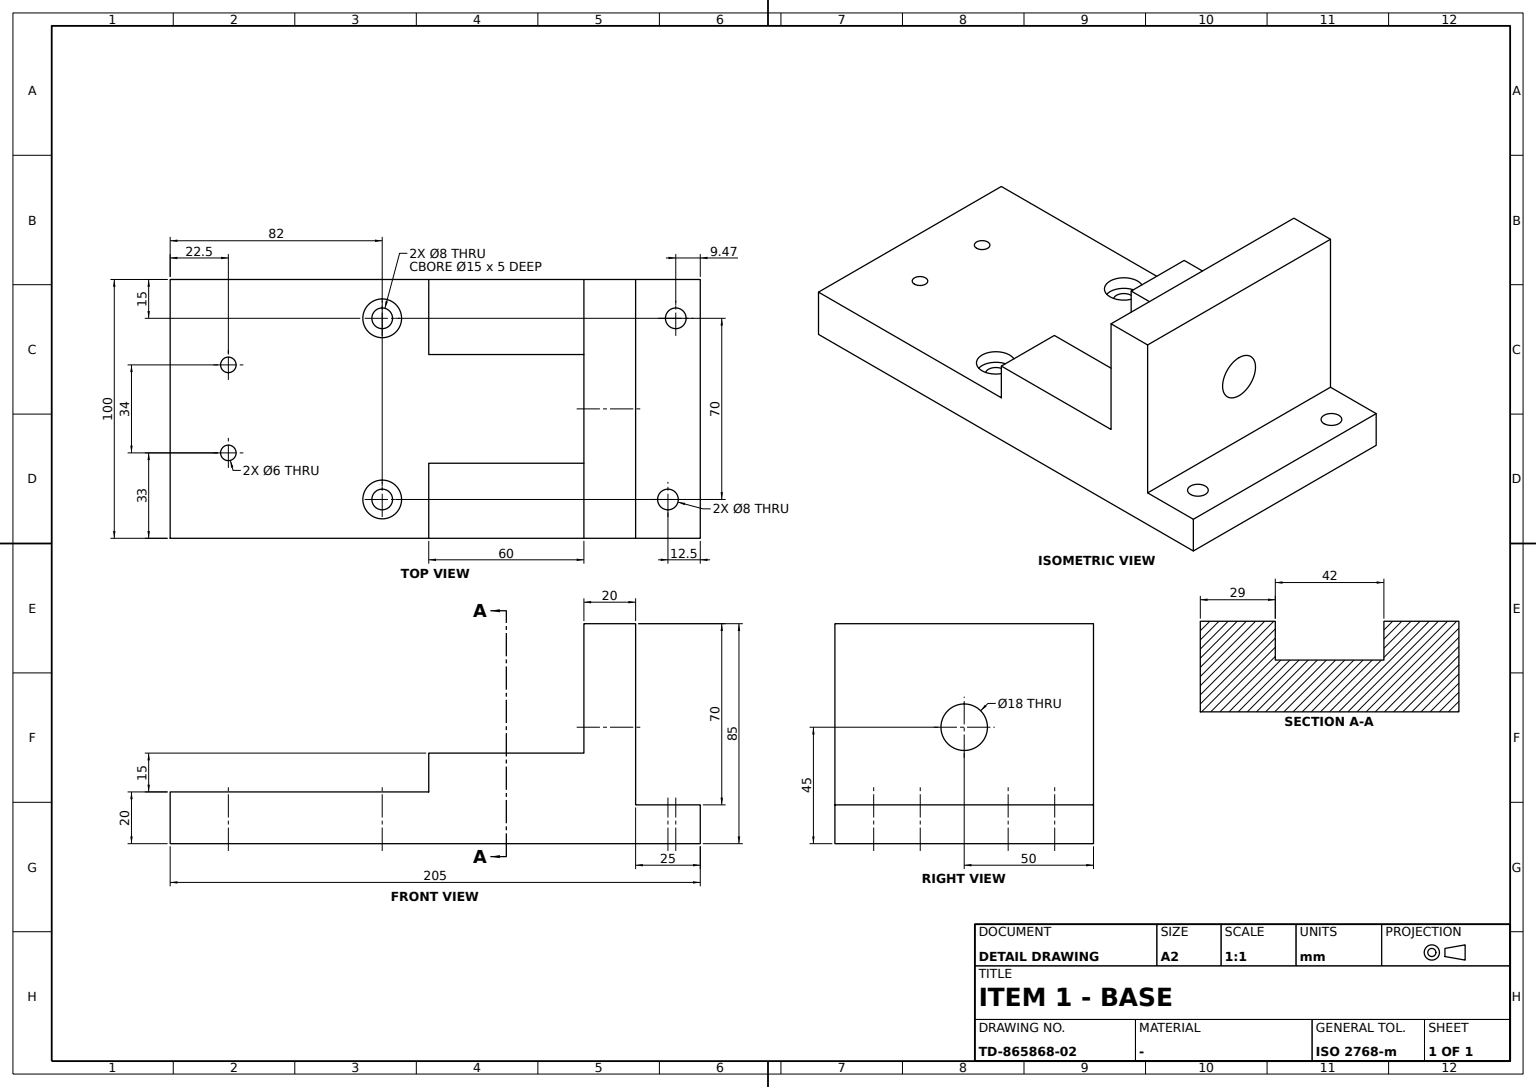
ISO-10303-21;
HEADER;
FILE_DESCRIPTION((''),'2;1');
FILE_NAME('','',(''),(''),'','','');
FILE_SCHEMA(('AUTOMOTIVE_DESIGN'));
ENDSEC;
DATA;
#1=APPLICATION_CONTEXT('');
#2=PRODUCT_CONTEXT('',#1,'mechanical');
#3=PRODUCT('','','',(#2));
#4=PRODUCT_DEFINITION_FORMATION('','',#3);
#5=PRODUCT_DEFINITION_CONTEXT('',#1,'design');
#6=PRODUCT_DEFINITION('','',#4,#5);
#7=PRODUCT_DEFINITION_SHAPE('','',#6);
#8=(LENGTH_UNIT()NAMED_UNIT(*)SI_UNIT(.MILLI.,.METRE.));
#9=(NAMED_UNIT(*)PLANE_ANGLE_UNIT()SI_UNIT($,.RADIAN.));
#10=(NAMED_UNIT(*)SI_UNIT($,.STERADIAN.)SOLID_ANGLE_UNIT());
#11=UNCERTAINTY_MEASURE_WITH_UNIT(LENGTH_MEASURE(0.005),#8,'distance_accuracy_value','');
#12=(GEOMETRIC_REPRESENTATION_CONTEXT(3)GLOBAL_UNCERTAINTY_ASSIGNED_CONTEXT((#11))GLOBAL_UNIT_ASSIGNED_CONTEXT((#8,#9,#10))REPRESENTATION_CONTEXT('',''));
#13=CARTESIAN_POINT('',(27.5,82.,15.));
#14=VERTEX_POINT('',#13);
#15=CARTESIAN_POINT('',(35.,82.,15.));
#16=DIRECTION('',(0.,0.,-1.));
#17=DIRECTION('',(-1.,0.,0.));
#18=AXIS2_PLACEMENT_3D('',#15,#16,#17);
#19=CIRCLE('',#18,7.5);
#20=EDGE_CURVE('',#14,#14,#19,.F.);
#21=ORIENTED_EDGE('',*,*,#20,.F.);
#22=EDGE_LOOP('',(#21));
#23=FACE_BOUND('',#22,.T.);
#24=CARTESIAN_POINT('',(27.5,82.,20.));
#25=VERTEX_POINT('',#24);
#26=CARTESIAN_POINT('',(35.,82.,20.));
#27=AXIS2_PLACEMENT_3D('',#26,#16,#17);
#28=CIRCLE('',#27,7.5);
#29=EDGE_CURVE('',#25,#25,#28,.F.);
#30=ORIENTED_EDGE('',*,*,#29,.T.);
#31=EDGE_LOOP('',(#30));
#32=FACE_BOUND('',#31,.T.);
#33=CARTESIAN_POINT('',(35.,82.,17.5));
#34=DIRECTION('',(0.,0.,1.));
#35=DIRECTION('',(0.,1.,0.));
#36=AXIS2_PLACEMENT_3D('',#33,#34,#35);
#37=CYLINDRICAL_SURFACE('',#36,7.5);
#38=ADVANCED_FACE('',(#23,#32),#37,.F.);
#39=CARTESIAN_POINT('',(-50.,160.,85.));
#40=VERTEX_POINT('',#39);
#41=CARTESIAN_POINT('',(50.,160.,85.));
#42=VERTEX_POINT('',#41);
#43=CARTESIAN_POINT('',(0.,160.,85.));
#44=DIRECTION('',(1.,0.,0.));
#45=VECTOR('',#44,1000.);
#46=LINE('',#43,#45);
#47=EDGE_CURVE('',#40,#42,#46,.T.);
#48=ORIENTED_EDGE('',*,*,#47,.T.);
#49=CARTESIAN_POINT('',(50.,180.,85.));
#50=VERTEX_POINT('',#49);
#51=CARTESIAN_POINT('',(50.,0.,85.));
#52=VECTOR('',#35,1000.);
#53=LINE('',#51,#52);
#54=EDGE_CURVE('',#42,#50,#53,.T.);
#55=ORIENTED_EDGE('',*,*,#54,.T.);
#56=CARTESIAN_POINT('',(-50.,180.,85.));
#57=VERTEX_POINT('',#56);
#58=CARTESIAN_POINT('',(0.,180.,85.));
#59=LINE('',#58,#45);
#60=EDGE_CURVE('',#57,#50,#59,.T.);
#61=ORIENTED_EDGE('',*,*,#60,.F.);
#62=CARTESIAN_POINT('',(-50.,0.,85.));
#63=LINE('',#62,#52);
#64=EDGE_CURVE('',#40,#57,#63,.T.);
#65=ORIENTED_EDGE('',*,*,#64,.F.);
#66=EDGE_LOOP('',(#48,#55,#61,#65));
#67=FACE_BOUND('',#66,.T.);
#68=AXIS2_PLACEMENT_3D('',#43,#16,#35);
#69=PLANE('',#68);
#70=ADVANCED_FACE('',(#67),#69,.F.);
#71=CARTESIAN_POINT('',(50.,100.,20.));
#72=VERTEX_POINT('',#71);
#73=CARTESIAN_POINT('',(21.,100.,20.));
#74=VERTEX_POINT('',#73);
#75=VECTOR('',#17,1000.);
#76=LINE('',#71,#75);
#77=EDGE_CURVE('',#72,#74,#76,.T.);
#78=ORIENTED_EDGE('',*,*,#77,.F.);
#79=CARTESIAN_POINT('',(50.,100.,35.));
#80=VERTEX_POINT('',#79);
#81=CARTESIAN_POINT('',(50.,100.,0.));
#82=VECTOR('',#34,1000.);
#83=LINE('',#81,#82);
#84=EDGE_CURVE('',#72,#80,#83,.T.);
#85=ORIENTED_EDGE('',*,*,#84,.T.);
#86=CARTESIAN_POINT('',(21.,100.,35.));
#87=VERTEX_POINT('',#86);
#88=CARTESIAN_POINT('',(0.,100.,35.));
#89=LINE('',#88,#75);
#90=EDGE_CURVE('',#80,#87,#89,.T.);
#91=ORIENTED_EDGE('',*,*,#90,.T.);
#92=LINE('',#73,#82);
#93=EDGE_CURVE('',#74,#87,#92,.T.);
#94=ORIENTED_EDGE('',*,*,#93,.F.);
#95=EDGE_LOOP('',(#78,#85,#91,#94));
#96=FACE_BOUND('',#95,.T.);
#97=AXIS2_PLACEMENT_3D('',#71,#35,#17);
#98=PLANE('',#97);
#99=ADVANCED_FACE('',(#96),#98,.F.);
#100=ORIENTED_EDGE('',*,*,#54,.F.);
#101=CARTESIAN_POINT('',(50.,160.,35.));
#102=VERTEX_POINT('',#101);
#103=CARTESIAN_POINT('',(50.,160.,0.));
#104=LINE('',#103,#82);
#105=EDGE_CURVE('',#102,#42,#104,.T.);
#106=ORIENTED_EDGE('',*,*,#105,.F.);
#107=CARTESIAN_POINT('',(50.,0.,35.));
#108=DIRECTION('',(0.,-1.,0.));
#109=VECTOR('',#108,1000.);
#110=LINE('',#107,#109);
#111=EDGE_CURVE('',#102,#80,#110,.T.);
#112=ORIENTED_EDGE('',*,*,#111,.T.);
#113=ORIENTED_EDGE('',*,*,#84,.F.);
#114=CARTESIAN_POINT('',(50.,0.,20.));
#115=VERTEX_POINT('',#114);
#116=LINE('',#114,#52);
#117=EDGE_CURVE('',#115,#72,#116,.T.);
#118=ORIENTED_EDGE('',*,*,#117,.F.);
#119=CARTESIAN_POINT('',(50.,0.,0.));
#120=VERTEX_POINT('',#119);
#121=LINE('',#119,#82);
#122=EDGE_CURVE('',#120,#115,#121,.T.);
#123=ORIENTED_EDGE('',*,*,#122,.F.);
#124=CARTESIAN_POINT('',(50.,205.,0.));
#125=VERTEX_POINT('',#124);
#126=LINE('',#119,#109);
#127=EDGE_CURVE('',#125,#120,#126,.T.);
#128=ORIENTED_EDGE('',*,*,#127,.F.);
#129=CARTESIAN_POINT('',(50.,205.,15.));
#130=VERTEX_POINT('',#129);
#131=VECTOR('',#16,1000.);
#132=LINE('',#124,#131);
#133=EDGE_CURVE('',#130,#125,#132,.T.);
#134=ORIENTED_EDGE('',*,*,#133,.F.);
#135=CARTESIAN_POINT('',(50.,180.,15.));
#136=VERTEX_POINT('',#135);
#137=CARTESIAN_POINT('',(50.,0.,15.));
#138=LINE('',#137,#52);
#139=EDGE_CURVE('',#136,#130,#138,.T.);
#140=ORIENTED_EDGE('',*,*,#139,.F.);
#141=CARTESIAN_POINT('',(50.,180.,0.));
#142=LINE('',#141,#131);
#143=EDGE_CURVE('',#50,#136,#142,.T.);
#144=ORIENTED_EDGE('',*,*,#143,.F.);
#145=EDGE_LOOP('',(#100,#106,#112,#113,#118,#123,#128,#134,#140,#144));
#146=FACE_BOUND('',#145,.T.);
#147=AXIS2_PLACEMENT_3D('',#119,#44,#35);
#148=PLANE('',#147);
#149=ADVANCED_FACE('',(#146),#148,.T.);
#150=CARTESIAN_POINT('',(-42.5,82.,15.));
#151=VERTEX_POINT('',#150);
#152=CARTESIAN_POINT('',(-35.,82.,15.));
#153=AXIS2_PLACEMENT_3D('',#152,#16,#17);
#154=CIRCLE('',#153,7.5);
#155=EDGE_CURVE('',#151,#151,#154,.F.);
#156=ORIENTED_EDGE('',*,*,#155,.F.);
#157=EDGE_LOOP('',(#156));
#158=FACE_BOUND('',#157,.T.);
#159=CARTESIAN_POINT('',(-42.5,82.,20.));
#160=VERTEX_POINT('',#159);
#161=CARTESIAN_POINT('',(-35.,82.,20.));
#162=AXIS2_PLACEMENT_3D('',#161,#16,#17);
#163=CIRCLE('',#162,7.5);
#164=EDGE_CURVE('',#160,#160,#163,.F.);
#165=ORIENTED_EDGE('',*,*,#164,.T.);
#166=EDGE_LOOP('',(#165));
#167=FACE_BOUND('',#166,.T.);
#168=CARTESIAN_POINT('',(-35.,82.,17.5));
#169=AXIS2_PLACEMENT_3D('',#168,#34,#35);
#170=CYLINDRICAL_SURFACE('',#169,7.5);
#171=ADVANCED_FACE('',(#158,#167),#170,.F.);
#172=CARTESIAN_POINT('',(-50.,180.,15.));
#173=VERTEX_POINT('',#172);
#174=CARTESIAN_POINT('',(0.,180.,15.));
#175=LINE('',#174,#45);
#176=EDGE_CURVE('',#173,#136,#175,.T.);
#177=ORIENTED_EDGE('',*,*,#176,.T.);
#178=ORIENTED_EDGE('',*,*,#139,.T.);
#179=CARTESIAN_POINT('',(-50.,205.,15.));
#180=VERTEX_POINT('',#179);
#181=CARTESIAN_POINT('',(0.,205.,15.));
#182=LINE('',#181,#45);
#183=EDGE_CURVE('',#180,#130,#182,.T.);
#184=ORIENTED_EDGE('',*,*,#183,.F.);
#185=CARTESIAN_POINT('',(-50.,0.,15.));
#186=LINE('',#185,#52);
#187=EDGE_CURVE('',#173,#180,#186,.T.);
#188=ORIENTED_EDGE('',*,*,#187,.F.);
#189=EDGE_LOOP('',(#177,#178,#184,#188));
#190=FACE_BOUND('',#189,.T.);
#191=CARTESIAN_POINT('',(-39.,195.52713,15.));
#192=VERTEX_POINT('',#191);
#193=CARTESIAN_POINT('',(-35.,195.52713,15.));
#194=AXIS2_PLACEMENT_3D('',#193,#16,#17);
#195=CIRCLE('',#194,4.);
#196=EDGE_CURVE('',#192,#192,#195,.T.);
#197=ORIENTED_EDGE('',*,*,#196,.T.);
#198=EDGE_LOOP('',(#197));
#199=FACE_BOUND('',#198,.T.);
#200=CARTESIAN_POINT('',(31.,192.5,15.));
#201=VERTEX_POINT('',#200);
#202=CARTESIAN_POINT('',(35.,192.5,15.));
#203=AXIS2_PLACEMENT_3D('',#202,#16,#17);
#204=CIRCLE('',#203,4.);
#205=EDGE_CURVE('',#201,#201,#204,.T.);
#206=ORIENTED_EDGE('',*,*,#205,.T.);
#207=EDGE_LOOP('',(#206));
#208=FACE_BOUND('',#207,.T.);
#209=AXIS2_PLACEMENT_3D('',#174,#16,#35);
#210=PLANE('',#209);
#211=ADVANCED_FACE('',(#190,#199,#208),#210,.F.);
#212=CARTESIAN_POINT('',(31.,82.,15.));
#213=VERTEX_POINT('',#212);
#214=CIRCLE('',#18,4.);
#215=EDGE_CURVE('',#213,#213,#214,.T.);
#216=ORIENTED_EDGE('',*,*,#215,.F.);
#217=EDGE_LOOP('',(#216));
#218=FACE_BOUND('',#217,.T.);
#219=CARTESIAN_POINT('',(39.,82.,0.));
#220=VERTEX_POINT('',#219);
#221=CARTESIAN_POINT('',(35.,82.,0.));
#222=AXIS2_PLACEMENT_3D('',#221,#34,#44);
#223=CIRCLE('',#222,4.);
#224=EDGE_CURVE('',#220,#220,#223,.T.);
#225=ORIENTED_EDGE('',*,*,#224,.F.);
#226=EDGE_LOOP('',(#225));
#227=FACE_BOUND('',#226,.T.);
#228=AXIS2_PLACEMENT_3D('',#15,#34,#35);
#229=CYLINDRICAL_SURFACE('',#228,4.);
#230=ADVANCED_FACE('',(#218,#227),#229,.F.);
#231=CARTESIAN_POINT('',(21.,160.,20.));
#232=VERTEX_POINT('',#231);
#233=CARTESIAN_POINT('',(21.,160.,35.));
#234=VERTEX_POINT('',#233);
#235=LINE('',#231,#82);
#236=EDGE_CURVE('',#232,#234,#235,.T.);
#237=ORIENTED_EDGE('',*,*,#236,.F.);
#238=LINE('',#73,#52);
#239=EDGE_CURVE('',#74,#232,#238,.T.);
#240=ORIENTED_EDGE('',*,*,#239,.F.);
#241=ORIENTED_EDGE('',*,*,#93,.T.);
#242=CARTESIAN_POINT('',(21.,0.,35.));
#243=LINE('',#242,#52);
#244=EDGE_CURVE('',#87,#234,#243,.T.);
#245=ORIENTED_EDGE('',*,*,#244,.T.);
#246=EDGE_LOOP('',(#237,#240,#241,#245));
#247=FACE_BOUND('',#246,.T.);
#248=AXIS2_PLACEMENT_3D('',#73,#44,#35);
#249=PLANE('',#248);
#250=ADVANCED_FACE('',(#247),#249,.F.);
#251=CARTESIAN_POINT('',(-21.,100.,20.));
#252=VERTEX_POINT('',#251);
#253=CARTESIAN_POINT('',(-21.,100.,35.));
#254=VERTEX_POINT('',#253);
#255=LINE('',#251,#82);
#256=EDGE_CURVE('',#252,#254,#255,.T.);
#257=ORIENTED_EDGE('',*,*,#256,.T.);
#258=CARTESIAN_POINT('',(-50.,100.,35.));
#259=VERTEX_POINT('',#258);
#260=LINE('',#79,#45);
#261=EDGE_CURVE('',#259,#254,#260,.T.);
#262=ORIENTED_EDGE('',*,*,#261,.F.);
#263=CARTESIAN_POINT('',(-50.,100.,20.));
#264=VERTEX_POINT('',#263);
#265=CARTESIAN_POINT('',(-50.,100.,0.));
#266=LINE('',#265,#82);
#267=EDGE_CURVE('',#264,#259,#266,.T.);
#268=ORIENTED_EDGE('',*,*,#267,.F.);
#269=CARTESIAN_POINT('',(0.,100.,20.));
#270=LINE('',#269,#45);
#271=EDGE_CURVE('',#264,#252,#270,.T.);
#272=ORIENTED_EDGE('',*,*,#271,.T.);
#273=EDGE_LOOP('',(#257,#262,#268,#272));
#274=FACE_BOUND('',#273,.T.);
#275=ADVANCED_FACE('',(#274),#98,.F.);
#276=CARTESIAN_POINT('',(0.,160.,35.));
#277=LINE('',#276,#45);
#278=EDGE_CURVE('',#234,#102,#277,.T.);
#279=ORIENTED_EDGE('',*,*,#278,.F.);
#280=ORIENTED_EDGE('',*,*,#244,.F.);
#281=ORIENTED_EDGE('',*,*,#90,.F.);
#282=ORIENTED_EDGE('',*,*,#111,.F.);
#283=EDGE_LOOP('',(#279,#280,#281,#282));
#284=FACE_BOUND('',#283,.T.);
#285=CARTESIAN_POINT('',(0.,0.,35.));
#286=AXIS2_PLACEMENT_3D('',#285,#34,#35);
#287=PLANE('',#286);
#288=ADVANCED_FACE('',(#284),#287,.T.);
#289=CARTESIAN_POINT('',(-14.,22.5,0.));
#290=VERTEX_POINT('',#289);
#291=CARTESIAN_POINT('',(-17.,22.5,0.));
#292=AXIS2_PLACEMENT_3D('',#291,#34,#44);
#293=CIRCLE('',#292,3.);
#294=EDGE_CURVE('',#290,#290,#293,.T.);
#295=ORIENTED_EDGE('',*,*,#294,.F.);
#296=EDGE_LOOP('',(#295));
#297=FACE_BOUND('',#296,.T.);
#298=CARTESIAN_POINT('',(-20.,22.5,20.));
#299=VERTEX_POINT('',#298);
#300=CARTESIAN_POINT('',(-17.,22.5,20.));
#301=AXIS2_PLACEMENT_3D('',#300,#16,#17);
#302=CIRCLE('',#301,3.);
#303=EDGE_CURVE('',#299,#299,#302,.T.);
#304=ORIENTED_EDGE('',*,*,#303,.F.);
#305=EDGE_LOOP('',(#304));
#306=FACE_BOUND('',#305,.T.);
#307=CARTESIAN_POINT('',(-17.,22.5,15.));
#308=AXIS2_PLACEMENT_3D('',#307,#34,#35);
#309=CYLINDRICAL_SURFACE('',#308,3.);
#310=ADVANCED_FACE('',(#297,#306),#309,.F.);
#311=CARTESIAN_POINT('',(39.,192.5,0.));
#312=VERTEX_POINT('',#311);
#313=CARTESIAN_POINT('',(35.,192.5,0.));
#314=AXIS2_PLACEMENT_3D('',#313,#34,#44);
#315=CIRCLE('',#314,4.);
#316=EDGE_CURVE('',#312,#312,#315,.T.);
#317=ORIENTED_EDGE('',*,*,#316,.T.);
#318=EDGE_LOOP('',(#317));
#319=FACE_BOUND('',#318,.T.);
#320=CARTESIAN_POINT('',(-31.,195.52713,0.));
#321=VERTEX_POINT('',#320);
#322=CARTESIAN_POINT('',(-35.,195.52713,0.));
#323=AXIS2_PLACEMENT_3D('',#322,#34,#44);
#324=CIRCLE('',#323,4.);
#325=EDGE_CURVE('',#321,#321,#324,.T.);
#326=ORIENTED_EDGE('',*,*,#325,.T.);
#327=EDGE_LOOP('',(#326));
#328=FACE_BOUND('',#327,.T.);
#329=ORIENTED_EDGE('',*,*,#127,.T.);
#330=CARTESIAN_POINT('',(-50.,0.,0.));
#331=VERTEX_POINT('',#330);
#332=CARTESIAN_POINT('',(0.,0.,0.));
#333=LINE('',#332,#45);
#334=EDGE_CURVE('',#331,#120,#333,.T.);
#335=ORIENTED_EDGE('',*,*,#334,.F.);
#336=CARTESIAN_POINT('',(-50.,205.,0.));
#337=VERTEX_POINT('',#336);
#338=LINE('',#330,#109);
#339=EDGE_CURVE('',#337,#331,#338,.T.);
#340=ORIENTED_EDGE('',*,*,#339,.F.);
#341=CARTESIAN_POINT('',(0.,205.,0.));
#342=LINE('',#341,#45);
#343=EDGE_CURVE('',#337,#125,#342,.T.);
#344=ORIENTED_EDGE('',*,*,#343,.T.);
#345=EDGE_LOOP('',(#329,#335,#340,#344));
#346=FACE_BOUND('',#345,.T.);
#347=ORIENTED_EDGE('',*,*,#294,.T.);
#348=EDGE_LOOP('',(#347));
#349=FACE_BOUND('',#348,.T.);
#350=CARTESIAN_POINT('',(20.,22.5,0.));
#351=VERTEX_POINT('',#350);
#352=CARTESIAN_POINT('',(17.,22.5,0.));
#353=AXIS2_PLACEMENT_3D('',#352,#34,#44);
#354=CIRCLE('',#353,3.);
#355=EDGE_CURVE('',#351,#351,#354,.T.);
#356=ORIENTED_EDGE('',*,*,#355,.T.);
#357=EDGE_LOOP('',(#356));
#358=FACE_BOUND('',#357,.T.);
#359=CARTESIAN_POINT('',(-31.,82.,0.));
#360=VERTEX_POINT('',#359);
#361=CARTESIAN_POINT('',(-35.,82.,0.));
#362=AXIS2_PLACEMENT_3D('',#361,#34,#44);
#363=CIRCLE('',#362,4.);
#364=EDGE_CURVE('',#360,#360,#363,.T.);
#365=ORIENTED_EDGE('',*,*,#364,.T.);
#366=EDGE_LOOP('',(#365));
#367=FACE_BOUND('',#366,.T.);
#368=ORIENTED_EDGE('',*,*,#224,.T.);
#369=EDGE_LOOP('',(#368));
#370=FACE_BOUND('',#369,.T.);
#371=AXIS2_PLACEMENT_3D('',#341,#34,#108);
#372=PLANE('',#371);
#373=ADVANCED_FACE('',(#319,#328,#346,#349,#358,#367,#370),#372,.F.);
#374=ORIENTED_EDGE('',*,*,#205,.F.);
#375=EDGE_LOOP('',(#374));
#376=FACE_BOUND('',#375,.T.);
#377=ORIENTED_EDGE('',*,*,#316,.F.);
#378=EDGE_LOOP('',(#377));
#379=FACE_BOUND('',#378,.T.);
#380=AXIS2_PLACEMENT_3D('',#202,#34,#35);
#381=CYLINDRICAL_SURFACE('',#380,4.);
#382=ADVANCED_FACE('',(#376,#379),#381,.F.);
#383=ORIENTED_EDGE('',*,*,#355,.F.);
#384=EDGE_LOOP('',(#383));
#385=FACE_BOUND('',#384,.T.);
#386=CARTESIAN_POINT('',(14.,22.5,20.));
#387=VERTEX_POINT('',#386);
#388=CARTESIAN_POINT('',(17.,22.5,20.));
#389=AXIS2_PLACEMENT_3D('',#388,#16,#17);
#390=CIRCLE('',#389,3.);
#391=EDGE_CURVE('',#387,#387,#390,.T.);
#392=ORIENTED_EDGE('',*,*,#391,.F.);
#393=EDGE_LOOP('',(#392));
#394=FACE_BOUND('',#393,.T.);
#395=CARTESIAN_POINT('',(17.,22.5,15.));
#396=AXIS2_PLACEMENT_3D('',#395,#34,#35);
#397=CYLINDRICAL_SURFACE('',#396,3.);
#398=ADVANCED_FACE('',(#385,#394),#397,.F.);
#399=CARTESIAN_POINT('',(-21.,160.,20.));
#400=VERTEX_POINT('',#399);
#401=LINE('',#399,#109);
#402=EDGE_CURVE('',#400,#252,#401,.T.);
#403=ORIENTED_EDGE('',*,*,#402,.F.);
#404=CARTESIAN_POINT('',(-21.,160.,35.));
#405=VERTEX_POINT('',#404);
#406=LINE('',#399,#82);
#407=EDGE_CURVE('',#400,#405,#406,.T.);
#408=ORIENTED_EDGE('',*,*,#407,.T.);
#409=CARTESIAN_POINT('',(-21.,0.,35.));
#410=LINE('',#409,#109);
#411=EDGE_CURVE('',#405,#254,#410,.T.);
#412=ORIENTED_EDGE('',*,*,#411,.T.);
#413=ORIENTED_EDGE('',*,*,#256,.F.);
#414=EDGE_LOOP('',(#403,#408,#412,#413));
#415=FACE_BOUND('',#414,.T.);
#416=AXIS2_PLACEMENT_3D('',#399,#17,#108);
#417=PLANE('',#416);
#418=ADVANCED_FACE('',(#415),#417,.F.);
#419=ORIENTED_EDGE('',*,*,#261,.T.);
#420=ORIENTED_EDGE('',*,*,#411,.F.);
#421=CARTESIAN_POINT('',(-50.,160.,35.));
#422=VERTEX_POINT('',#421);
#423=LINE('',#276,#75);
#424=EDGE_CURVE('',#422,#405,#423,.F.);
#425=ORIENTED_EDGE('',*,*,#424,.F.);
#426=CARTESIAN_POINT('',(-50.,0.,35.));
#427=LINE('',#426,#52);
#428=EDGE_CURVE('',#259,#422,#427,.T.);
#429=ORIENTED_EDGE('',*,*,#428,.F.);
#430=EDGE_LOOP('',(#419,#420,#425,#429));
#431=FACE_BOUND('',#430,.T.);
#432=ADVANCED_FACE('',(#431),#287,.T.);
#433=ORIENTED_EDGE('',*,*,#343,.F.);
#434=LINE('',#336,#131);
#435=EDGE_CURVE('',#180,#337,#434,.T.);
#436=ORIENTED_EDGE('',*,*,#435,.F.);
#437=ORIENTED_EDGE('',*,*,#183,.T.);
#438=ORIENTED_EDGE('',*,*,#133,.T.);
#439=EDGE_LOOP('',(#433,#436,#437,#438));
#440=FACE_BOUND('',#439,.T.);
#441=AXIS2_PLACEMENT_3D('',#181,#108,#16);
#442=PLANE('',#441);
#443=ADVANCED_FACE('',(#440),#442,.F.);
#444=CARTESIAN_POINT('',(0.,160.,54.));
#445=VERTEX_POINT('',#444);
#446=CARTESIAN_POINT('',(0.,160.,45.));
#447=AXIS2_PLACEMENT_3D('',#446,#35,#34);
#448=CIRCLE('',#447,9.);
#449=EDGE_CURVE('',#445,#445,#448,.T.);
#450=ORIENTED_EDGE('',*,*,#449,.T.);
#451=EDGE_LOOP('',(#450));
#452=FACE_BOUND('',#451,.T.);
#453=CARTESIAN_POINT('',(-50.,160.,0.));
#454=LINE('',#453,#82);
#455=EDGE_CURVE('',#422,#40,#454,.T.);
#456=ORIENTED_EDGE('',*,*,#455,.F.);
#457=ORIENTED_EDGE('',*,*,#424,.T.);
#458=ORIENTED_EDGE('',*,*,#407,.F.);
#459=CARTESIAN_POINT('',(0.,160.,20.));
#460=LINE('',#459,#45);
#461=EDGE_CURVE('',#400,#232,#460,.T.);
#462=ORIENTED_EDGE('',*,*,#461,.T.);
#463=ORIENTED_EDGE('',*,*,#236,.T.);
#464=ORIENTED_EDGE('',*,*,#278,.T.);
#465=ORIENTED_EDGE('',*,*,#105,.T.);
#466=ORIENTED_EDGE('',*,*,#47,.F.);
#467=EDGE_LOOP('',(#456,#457,#458,#462,#463,#464,#465,#466));
#468=FACE_BOUND('',#467,.T.);
#469=AXIS2_PLACEMENT_3D('',#459,#35,#34);
#470=PLANE('',#469);
#471=ADVANCED_FACE('',(#452,#468),#470,.F.);
#472=CARTESIAN_POINT('',(0.,180.,36.));
#473=VERTEX_POINT('',#472);
#474=CARTESIAN_POINT('',(0.,180.,45.));
#475=AXIS2_PLACEMENT_3D('',#474,#108,#16);
#476=CIRCLE('',#475,9.);
#477=EDGE_CURVE('',#473,#473,#476,.F.);
#478=ORIENTED_EDGE('',*,*,#477,.F.);
#479=EDGE_LOOP('',(#478));
#480=FACE_BOUND('',#479,.T.);
#481=CARTESIAN_POINT('',(-50.,180.,0.));
#482=LINE('',#481,#131);
#483=EDGE_CURVE('',#57,#173,#482,.T.);
#484=ORIENTED_EDGE('',*,*,#483,.F.);
#485=ORIENTED_EDGE('',*,*,#60,.T.);
#486=ORIENTED_EDGE('',*,*,#143,.T.);
#487=ORIENTED_EDGE('',*,*,#176,.F.);
#488=EDGE_LOOP('',(#484,#485,#486,#487));
#489=FACE_BOUND('',#488,.T.);
#490=AXIS2_PLACEMENT_3D('',#58,#108,#16);
#491=PLANE('',#490);
#492=ADVANCED_FACE('',(#480,#489),#491,.F.);
#493=ORIENTED_EDGE('',*,*,#20,.T.);
#494=EDGE_LOOP('',(#493));
#495=FACE_BOUND('',#494,.T.);
#496=ORIENTED_EDGE('',*,*,#215,.T.);
#497=EDGE_LOOP('',(#496));
#498=FACE_BOUND('',#497,.T.);
#499=ADVANCED_FACE('',(#495,#498),#210,.F.);
#500=CARTESIAN_POINT('',(-50.,0.,20.));
#501=VERTEX_POINT('',#500);
#502=LINE('',#330,#82);
#503=EDGE_CURVE('',#331,#501,#502,.T.);
#504=ORIENTED_EDGE('',*,*,#503,.F.);
#505=ORIENTED_EDGE('',*,*,#334,.T.);
#506=ORIENTED_EDGE('',*,*,#122,.T.);
#507=CARTESIAN_POINT('',(0.,0.,20.));
#508=LINE('',#507,#45);
#509=EDGE_CURVE('',#501,#115,#508,.T.);
#510=ORIENTED_EDGE('',*,*,#509,.F.);
#511=EDGE_LOOP('',(#504,#505,#506,#510));
#512=FACE_BOUND('',#511,.T.);
#513=AXIS2_PLACEMENT_3D('',#332,#35,#34);
#514=PLANE('',#513);
#515=ADVANCED_FACE('',(#512),#514,.F.);
#516=ORIENTED_EDGE('',*,*,#477,.T.);
#517=EDGE_LOOP('',(#516));
#518=FACE_BOUND('',#517,.T.);
#519=ORIENTED_EDGE('',*,*,#449,.F.);
#520=EDGE_LOOP('',(#519));
#521=FACE_BOUND('',#520,.T.);
#522=CARTESIAN_POINT('',(0.,155.,45.));
#523=AXIS2_PLACEMENT_3D('',#522,#35,#17);
#524=CYLINDRICAL_SURFACE('',#523,9.);
#525=ADVANCED_FACE('',(#518,#521),#524,.F.);
#526=ORIENTED_EDGE('',*,*,#303,.T.);
#527=EDGE_LOOP('',(#526));
#528=FACE_BOUND('',#527,.T.);
#529=ORIENTED_EDGE('',*,*,#29,.F.);
#530=EDGE_LOOP('',(#529));
#531=FACE_BOUND('',#530,.T.);
#532=ORIENTED_EDGE('',*,*,#391,.T.);
#533=EDGE_LOOP('',(#532));
#534=FACE_BOUND('',#533,.T.);
#535=ORIENTED_EDGE('',*,*,#164,.F.);
#536=EDGE_LOOP('',(#535));
#537=FACE_BOUND('',#536,.T.);
#538=ORIENTED_EDGE('',*,*,#461,.F.);
#539=ORIENTED_EDGE('',*,*,#402,.T.);
#540=ORIENTED_EDGE('',*,*,#271,.F.);
#541=LINE('',#500,#52);
#542=EDGE_CURVE('',#501,#264,#541,.T.);
#543=ORIENTED_EDGE('',*,*,#542,.F.);
#544=ORIENTED_EDGE('',*,*,#509,.T.);
#545=ORIENTED_EDGE('',*,*,#117,.T.);
#546=ORIENTED_EDGE('',*,*,#77,.T.);
#547=ORIENTED_EDGE('',*,*,#239,.T.);
#548=EDGE_LOOP('',(#538,#539,#540,#543,#544,#545,#546,#547));
#549=FACE_BOUND('',#548,.T.);
#550=AXIS2_PLACEMENT_3D('',#507,#16,#35);
#551=PLANE('',#550);
#552=ADVANCED_FACE('',(#528,#531,#534,#537,#549),#551,.F.);
#553=ORIENTED_EDGE('',*,*,#325,.F.);
#554=EDGE_LOOP('',(#553));
#555=FACE_BOUND('',#554,.T.);
#556=ORIENTED_EDGE('',*,*,#196,.F.);
#557=EDGE_LOOP('',(#556));
#558=FACE_BOUND('',#557,.T.);
#559=AXIS2_PLACEMENT_3D('',#193,#34,#35);
#560=CYLINDRICAL_SURFACE('',#559,4.);
#561=ADVANCED_FACE('',(#555,#558),#560,.F.);
#562=CARTESIAN_POINT('',(-39.,82.,15.));
#563=VERTEX_POINT('',#562);
#564=CIRCLE('',#153,4.);
#565=EDGE_CURVE('',#563,#563,#564,.T.);
#566=ORIENTED_EDGE('',*,*,#565,.T.);
#567=EDGE_LOOP('',(#566));
#568=FACE_BOUND('',#567,.T.);
#569=ORIENTED_EDGE('',*,*,#155,.T.);
#570=EDGE_LOOP('',(#569));
#571=FACE_BOUND('',#570,.T.);
#572=ADVANCED_FACE('',(#568,#571),#210,.F.);
#573=ORIENTED_EDGE('',*,*,#542,.T.);
#574=ORIENTED_EDGE('',*,*,#267,.T.);
#575=ORIENTED_EDGE('',*,*,#428,.T.);
#576=ORIENTED_EDGE('',*,*,#455,.T.);
#577=ORIENTED_EDGE('',*,*,#64,.T.);
#578=ORIENTED_EDGE('',*,*,#483,.T.);
#579=ORIENTED_EDGE('',*,*,#187,.T.);
#580=ORIENTED_EDGE('',*,*,#435,.T.);
#581=ORIENTED_EDGE('',*,*,#339,.T.);
#582=ORIENTED_EDGE('',*,*,#503,.T.);
#583=EDGE_LOOP('',(#573,#574,#575,#576,#577,#578,#579,#580,#581,#582));
#584=FACE_BOUND('',#583,.T.);
#585=AXIS2_PLACEMENT_3D('',#330,#44,#35);
#586=PLANE('',#585);
#587=ADVANCED_FACE('',(#584),#586,.F.);
#588=ORIENTED_EDGE('',*,*,#364,.F.);
#589=EDGE_LOOP('',(#588));
#590=FACE_BOUND('',#589,.T.);
#591=ORIENTED_EDGE('',*,*,#565,.F.);
#592=EDGE_LOOP('',(#591));
#593=FACE_BOUND('',#592,.T.);
#594=AXIS2_PLACEMENT_3D('',#152,#34,#35);
#595=CYLINDRICAL_SURFACE('',#594,4.);
#596=ADVANCED_FACE('',(#590,#593),#595,.F.);
#597=CLOSED_SHELL('',(#38,#70,#99,#149,#171,#211,#230,#250,#275,#288,#310,#373,#382,#398,#418,#432,#443,#471,#492,#499,#515,#525,#552,#561,#572,#587,#596));
#598=MANIFOLD_SOLID_BREP('',#597);
#599=ADVANCED_BREP_SHAPE_REPRESENTATION('',(#598),#12);
#600=SHAPE_DEFINITION_REPRESENTATION(#7,#599);
ENDSEC;
END-ISO-10303-21;
